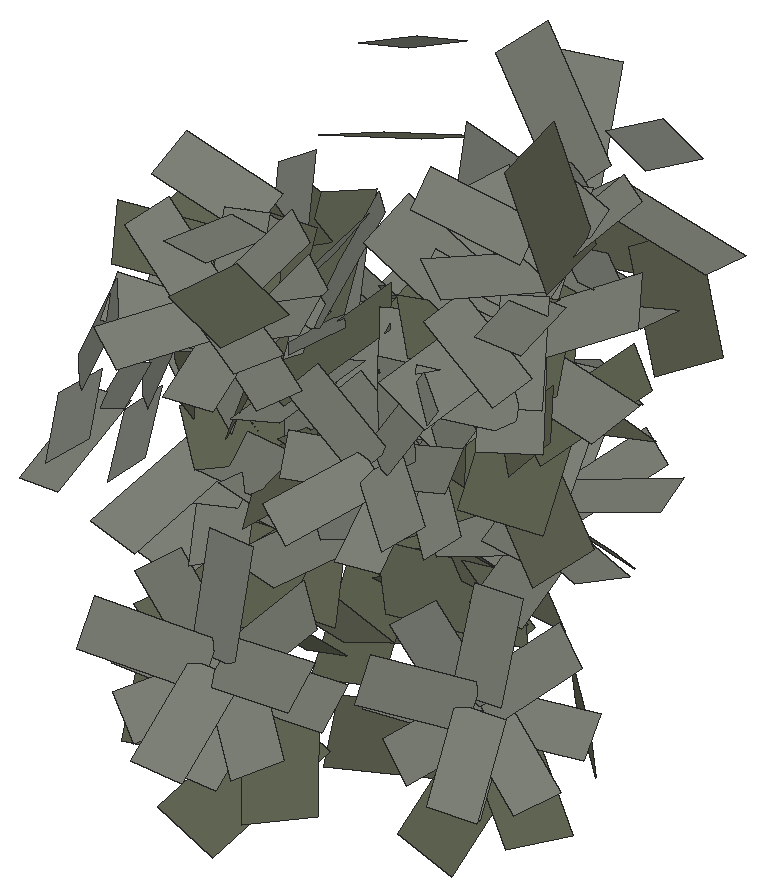
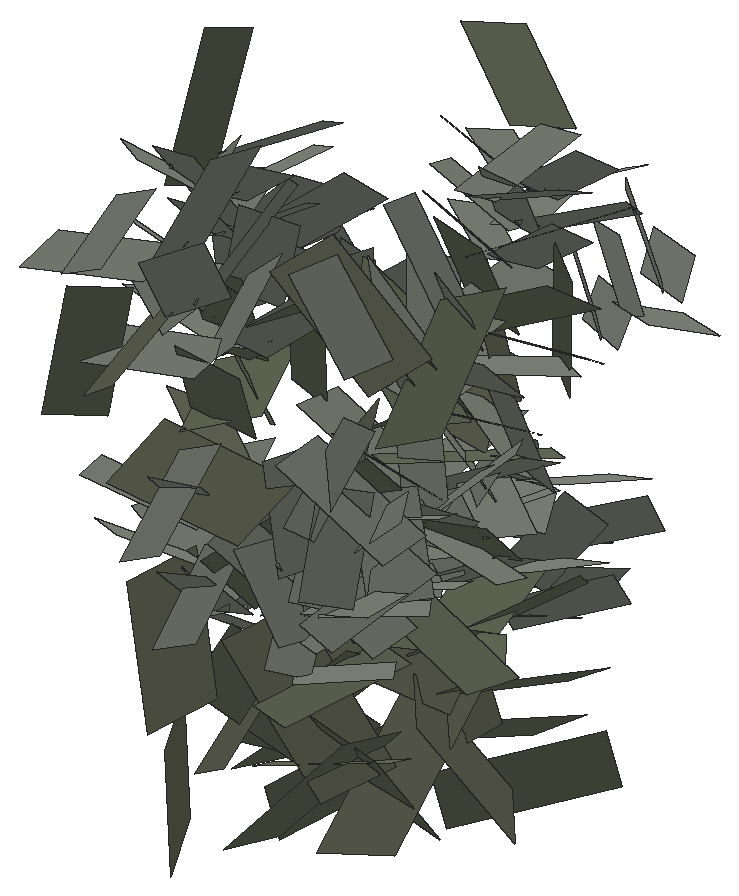
# SketchUp Ruby script. Lengths in inches.
U = 1.inch
M = Sketchup.active_model
def pt(a) = Geom::Point3d.new(a.map { |v| v * U })
def face(e, loops, mat)
  f = e.add_face(loops[0].map { |a| pt(a) })
  loops[1..].each { |l| e.add_face(l.map { |a| pt(a) }).erase! }
  f.material = f.back_material = mat if mat
  f
end
# faces: each face lists its corners as indices into pts; further lists are holes
def faces(e, pts, list, mat = nil) = list.each { |f| face(e, (f[0].is_a?(Array) ? f : [f]).map { |l| l.map { |i| pts[i] } }, mat) }
# xy, xz, yz: faces in a plane at the given z, y or x. An outline is a flat list of corners, or four numbers for a rectangle; further outlines are holes
def ring(l) = l.size == 4 ? [[l[0], l[1]], [l[2], l[1]], [l[2], l[3]], [l[0], l[3]]] : l.each_slice(2).to_a
def flat(e, list, mat, &to3) = list.each { |f| face(e, (f[0].is_a?(Array) ? f : [f]).map { |l| ring(l).map { |u, v| to3.(u, v) } }, mat) }
def xy(e, z, list, mat = nil) = flat(e, list, mat) { |x, y| [x, y, z] }
def xz(e, y, list, mat = nil) = flat(e, list, mat) { |x, z| [x, y, z] }
def yz(e, x, list, mat = nil) = flat(e, list, mat) { |y, z| [x, y, z] }
def lines(e, pts, list) = list.each { |a, b| e.add_line(pt(pts[a]), pt(pts[b])) }
# prism: a flat outline (further loops are holes) pulled along v
def prism(e, loops, v, mat = nil)
  f = face(e, loops, mat); d = Geom::Vector3d.new(v.map { |x| x * U })
  f.pushpull(f.normal.samedirection?(d) ? d.length : -d.length)
end
def box(e, o, s, mat = nil) = prism(e, [[o, [o[0] + s[0], o[1], o[2]], [o[0] + s[0], o[1] + s[1], o[2]], [o[0], o[1] + s[1], o[2]]]], [0, 0, s[2]], mat)
def at(x, y, z, deg = 0) = Geom::Transformation.translation(pt([x, y, z])) * Geom::Transformation.rotation(ORIGIN, Z_AXIS, deg.degrees)
def axes(o, x, y, z) = Geom::Transformation.new([*x, 0, *y, 0, *z, 0, *pt(o).to_a, 1])
def part(name) = M.definitions.add(name)
# library, detail: a bought-in or finely detailed component or shape, given as its bounding box
def library(name, o, s) = part(name).tap { |d| box(d.entities, o, s) }
def detail(e, o, s) = box(e.add_group.entities, o, s)
def put(e, d, t, mat = nil) = e.add_instance(d, t).tap { |i| i.material = mat if mat }
def group(e, t, mat = nil) = e.add_group.tap { |g| g.transformation = t; g.material = mat if mat }.entities
root = M.entities
M.materials.add("viburnumblaasdfas0df1w06d").color = [98, 102, 84]
M.materials.add("viburnumbladsadfasdfad0w122").color = [125, 129, 119]
c1 = part("Component\#315")
p = [[0.25,0,0],[2.05,0.01,0.35],[1.81,4.2,1.66],[0,4.19,1.3125]]
faces(c1.entities,p,[[0,1,2,3]],"viburnumbladsadfasdfad0w122")
c2 = part("viburnumblad2")
put(c2.entities,c1,axes([-19.23,-4.49,-32.18],[83.35428,0,0],[0,79.38502,0],[0,0,83.35428]))
c3 = part("Component\#314")
p = [[0.14,0,0],[2.58,0.05,0.25],[2.44,5.11,2.64],[0,5.05,2.39]]
faces(c3.entities,p,[[0,1,2,3]],"viburnumblaasdfas0df1w06d")
c4 = part("viburnumblad1\#2")
put(c4.entities,c3,axes([-37.25,6.23,19.31],[75.98784,0,0],[0,65.50676,0],[0,0,75.98784]))
put(root,c2,axes([1229.08,191.18,23.91],[-0.00766,-0.00322,-0.00823],[0.00764,-0.00813,-0.00386],[-0.0046,-0.00755,0.00633]))
put(root,c2,axes([1229.875,191.74,22.7],[-0.01118,0.00278,-0.00257],[-0.00011,-0.00839,-0.00838],[-0.00365,-0.00753,0.00688]))
put(root,c4,axes([1233.54,192.86,28.38],[-0.00662,-0.01127,-0.00498],[0.01432,-0.00702,-0.0031],[-0.00011,-0.00548,0.01154]))
put(root,c2,axes([1233.59,192.42,26.27],[-0.00995,0.00489,0.00397],[-0.00607,-0.00954,-0.00338],[0.0019,-0.00477,0.00949]))
put(root,c2,axes([1233.79,193.03,12.62],[-0.01241,-0.00141,0.00136],[-0.00002,-0.00862,-0.00914],[0.00196,-0.00903,0.00851]))
put(root,c2,axes([1227.68,191.68,23.79],[0.00814,-0.00715,-0.0046],[0.00716,0.00216,0.00888],[-0.00455,-0.00881,0.00477]))
put(root,c2,axes([1228.74,192.77,23.34],[0.00034,-0.00733,-0.00907],[0.00978,-0.00348,0.00299],[-0.00497,-0.00808,0.00546]))
put(root,c2,axes([1229.97,193.27,22.62],[-0.00655,-0.0022,-0.00816],[0.00764,-0.00813,-0.00386],[-0.0054,-0.00785,0.00541]))
put(root,c2,axes([1233.84,193.93,25.53],[-0.01146,-0.00283,-0.00038],[0.00275,-0.01049,-0.00491],[0.00082,-0.00467,0.00968]))
put(root,c2,axes([1233.51,193.6875,27.03],[-0.00626,-0.00889,-0.00451],[0.01001,-0.00557,-0.00285],[-0.00007,-0.00526,0.00943]))
put(root,c2,axes([1232.49,192.34,12.02],[0.00026,0.00745,0.01011],[-0.01208,-0.00262,0.00224],[0.00344,-0.00977,0.00711]))
put(root,c2,axes([1233.23,193.92,11.1875],[-0.00859,0.00427,0.00811],[-0.00794,-0.00683,-0.00482],[0.00302,-0.00917,0.00803]))
put(root,c2,axes([1232.85,192.9,25.04],[-0.00261,0.00974,0.006],[-0.01123,-0.00353,0.00072],[0.00254,-0.00551,0.00899]))
put(root,c2,axes([1232.92,193.69,13.76],[-0.00026,-0.00745,-0.01011],[0.01255,0.00018,-0.00046],[0.00042,-0.01011,0.00745]))
put(root,c2,axes([1233.14,194.77,12.4],[-0.00896,-0.00627,-0.00619],[0.0092,-0.00573,-0.00751],[0.00088,-0.00942,0.00827]))
put(root,c2,axes([1228.8,193.73,22.42],[0.0085,-0.00746,-0.0048],[0.00645,0.00195,0.00799],[-0.00455,-0.00881,0.00477]))
put(root,c2,axes([1232.1,192.27,26.35],[0.00626,0.00889,0.00451],[-0.00973,0.00413,0.00504],[0.00235,-0.00645,0.00846]))
put(root,c2,axes([1233.23,195.2,24.93],[-0.00572,-0.00761,-0.00506],[0.01001,-0.00557,-0.00285],[-0.00075,-0.00619,0.00889]))
put(root,c2,axes([1233.15,195.37,10.67],[-0.01296,-0.00148,0.00142],[-0.00002,-0.00776,-0.00823],[0.00196,-0.00903,0.00851]))
put(root,c2,axes([1231.62,193,13.17],[0.01241,0.00141,-0.00136],[0.00049,0.00618,0.01093],[0.0019,-0.01085,0.00605]))
put(root,c2,axes([1238.62,194.75,20.89],[-0.00871,0.00384,0.00541],[-0.00663,-0.00614,-0.00616],[0.00084,-0.00787,0.00624]))
put(root,c2,axes([1232.43,194.64,26.07],[0.00261,-0.00974,-0.006],[0.01057,0.00192,0.00135],[-0.00026,-0.0062,0.0089]))
put(root,c2,axes([1238.67,195.56,22],[-0.00668,-0.00514,-0.00687],[0.00865,-0.00485,-0.0047],[-0.00103,-0.00803,0.00606]))
put(root,c2,axes([1231.48,193.69,11.4],[0.00896,0.00627,0.00619],[-0.00837,0.00305,0.00903],[0.00298,-0.01046,0.00629]))
put(root,c2,axes([1232.03,193.55,27.11],[0.00995,-0.00489,-0.00397],[0.00635,0.0081,0.00558],[0.00038,-0.00694,0.0084]))
put(root,c2,axes([1232.09,194.68,10.17],[-0.00011,0.00779,0.00854],[-0.01208,-0.00262,0.00224],[0.00345,-0.0089,0.00816]))
put(root,c2,axes([1233.05,196.87,28.49],[-0.01199,0.00073,-0.00108],[-0.00063,-0.01339,-0.00213],[-0.00123,-0.0019,0.01236]))
put(root,c2,axes([1239.06,196.29,20.8125],[-0.01089,-0.00092,-0.00104],[0.00144,-0.00742,-0.00803],[-0.00015,-0.00772,0.00646]))
put(root,c2,axes([1231.75,194.66,12.66],[0.00859,-0.00427,-0.00811],[0.00913,0.005,0.00703],[0.00084,-0.0107,0.00653]))
put(root,c2,axes([1232.17,193.83,24.1],[0.00601,0.00853,0.00433],[-0.01051,0.00446,0.00545],[0.00235,-0.00645,0.00846]))
put(root,c2,axes([1231.79,193.55,25.51],[0.01146,0.00283,0.00038],[-0.00257,0.0094,0.00741],[0.00146,-0.00704,0.00821]))
put(root,c2,axes([1230.12,196.91,17.89],[-0.01312,0.00207,0.00149],[-0.00255,-0.01047,-0.0079],[-0.00005,-0.00804,0.01068]))
put(root,c2,axes([1232.14,196.01,11.74],[-0.00025,-0.00716,-0.0097],[0.01356,0.0002,-0.00049],[0.00042,-0.01011,0.00745]))
put(root,c2,axes([1237.23,194.77,20.95],[0.00668,0.00514,0.00687],[-0.00864,0.00277,0.00603],[0.00109,-0.00897,0.00475]))
put(root,c4,axes([1232.7,198.28,9.32],[-0.01126,-0.00753,-0.00255],[0.00827,-0.00884,-0.01044],[0.00351,-0.00867,0.01012]))
put(root,c4,axes([1229.32,195.73,20.55],[0.01089,-0.00679,0.00142],[0.00218,0.00667,0.0129],[-0.00665,-0.00902,0.00468]))
put(root,c4,axes([1232.75,196.73,25.15],[-0.0066,0.01089,0.00527],[-0.0139,-0.00777,-0.00135],[0.00164,-0.00514,0.01268]))
put(root,c2,axes([1238.04,195.71,20.04],[-0.00143,0.00635,0.00868],[-0.0108,-0.00196,-0.00037],[0.00136,-0.00839,0.00553]))
put(root,c2,axes([1237.29,195.58,22.05],[0.00871,-0.00384,-0.00541],[0.00664,0.00406,0.00749],[-0.00079,-0.00912,0.00457]))
put(root,c2,axes([1231.97,195.07,24.9],[0.01038,-0.0051,-0.00415],[0.00572,0.00729,0.00502],[0.00038,-0.00694,0.0084]))
put(root,c4,axes([1232.74,198.97,19.44],[-0.00918,-0.00626,-0.00848],[0.01129,-0.01094,-0.00412],[-0.00395,-0.00772,0.00939]))
put(root,c4,axes([1230.57,197.7,20.49],[0.00428,-0.01029,-0.00658],[0.01194,-0.00078,0.00879],[-0.00649,-0.00737,0.00685]))
put(root,c2,axes([1237.83,196.86,21.56],[0.00143,-0.00635,-0.00868],[0.00992,-0.00012,0.00155],[-0.0013,-0.00861,0.00528]))
put(root,c4,axes([1232.6,199.28,6.97],[-0.01186,-0.00066,0.00699],[-0.00532,-0.01121,-0.01007],[0.00532,-0.0098,0.0081]))
put(root,c2,axes([1232.3,198.48,24.74],[-0.01244,-0.00019,-0.00567],[0.00199,-0.01294,-0.00394],[-0.00531,-0.00441,0.0118]))
put(root,c2,axes([1238.68,197.67,20.78],[-0.00601,-0.0039,-0.00689],[0.00865,-0.00485,-0.0047],[-0.00175,-0.00854,0.00529]))
put(root,c2,axes([1229.42,198.03,18.94],[-0.00252,-0.00942,-0.00914],[0.01298,-0.00318,-0.00031],[-0.00196,-0.00893,0.00974]))
put(root,c2,axes([1229.9,198.8,17.3125],[-0.01106,-0.0052,-0.00541],[0.00776,-0.00965,-0.0066],[-0.00127,-0.0082,0.01048]))
put(root,c2,axes([1231.8,195.9375,28.14],[0.00044,0.0126,0.00361],[-0.0113,0.00031,0.00032],[0.00024,-0.00347,0.01207]))
put(root,c2,axes([1240.93,198.61,11.125],[-0.01026,-0.00498,0.00256],[0.0015,-0.00759,-0.00876],[0.0054,-0.00736,0.0073]))
put(root,c2,axes([1239.93,197.61,10.69],[-0.00083,0.00664,0.00958],[-0.0095,-0.00594,0.0033],[0.00675,-0.00756,0.00582]))
put(root,c2,axes([1237.125,196.21,20.71],[0.01089,0.00092,0.00104],[-0.00149,0.00552,0.00975],[0.0002,-0.00927,0.00435]))
put(root,c4,axes([1231.34,196.125,22.41],[0.01287,-0.00107,0.00071],[0.00034,0.01171,0.00907],[-0.00141,-0.0079,0.00892]))
put(root,c4,axes([1232.83,199.58,19.46],[-0.00628,-0.01206,-0.00336],[0.01448,-0.00668,-0.00311],[0.00091,-0.00388,0.01211]))
put(root,c2,axes([1233.52,199.6,17.84],[-0.01428,0.00021,0.00102],[-0.00037,-0.01414,-0.00224],[0.00098,-0.00226,0.01411]))
put(root,c2,axes([1230,199.08,15.39],[-0.0137,0.00216,0.00156],[-0.00229,-0.00943,-0.00711],[-0.00005,-0.00804,0.01068]))
put(root,c2,axes([1237.56,196.9375,19.61],[0.00642,0.00493,0.0066],[-0.00933,0.00299,0.00651],[0.00109,-0.00897,0.00475]))
put(root,c2,axes([1241.58,198.21,22.68],[-0.00449,0.00779,0.00619],[-0.00867,-0.00648,0.00177],[0.0049,-0.00408,0.00781]))
put(root,c2,axes([1232.61,198.76,22.875],[-0.01065,0.00857,-0.00023],[-0.00787,-0.00997,-0.00669],[-0.00415,-0.00484,0.01209]))
put(root,c2,axes([1240,199.22,9.9],[-0.00784,0.00117,0.00859],[-0.00546,-0.0084,-0.00383],[0.00631,-0.00716,0.00674]))
put(root,c2,axes([1237.49,197.72,20.74],[0.00909,-0.00401,-0.00564],[0.00597,0.00365,0.00674],[-0.00079,-0.00912,0.00457]))
put(root,c2,axes([1240.67,200,24.8],[-0.01366,0.00095,0.00535],[-0.00336,-0.01286,-0.00628],[0.00428,-0.00706,0.01216]))
put(root,c2,axes([1233.24,200.25,21.93],[-0.01194,-0.00018,-0.00545],[0.00215,-0.01397,-0.00426],[-0.00531,-0.00441,0.0118]))
put(root,c2,axes([1232.42,200.14,23.55],[-0.00694,-0.00883,-0.00779],[0.00996,-0.00923,0.0016],[-0.00629,-0.00487,0.01112]))
put(root,c4,axes([1231.67,197.14,22.86],[0.0051,0.011,0.00655],[-0.01483,0.00551,0.0023],[-0.00067,-0.00681,0.01196]))
put(root,c2,axes([1241.27,197.43,23.96],[0.00334,0.0097,0.00381],[-0.00915,0.00071,0.00588],[0.00496,-0.00497,0.00731]))
put(root,c2,axes([1231.21,197.57,23.76],[-0.00263,0.0123,0.00535],[-0.01296,-0.00091,-0.00426],[-0.00348,-0.00589,0.01184]))
put(root,c4,axes([1231.57,198.18,21.39],[0.0077,-0.00971,-0.00377],[0.01191,0.00736,0.00523],[-0.00177,-0.00557,0.01033]))
put(root,c2,axes([1233,200.9,14.51],[-0.01371,0.0002,0.00098],[-0.0004,-0.01527,-0.00242],[0.00098,-0.00226,0.01411]))
put(root,c4,axes([1230.25,201.88,13.42],[-0.01365,-0.00518,-0.0014],[0.0059,-0.01311,-0.00908],[0.00168,-0.00777,0.01232]))
put(root,c2,axes([1227.89,197.56,18.43],[0.01312,-0.00207,-0.00149],[0.00246,0.00822,0.01025],[-0.00067,-0.01033,0.00845]))
put(root,c2,axes([1232.86,199.58,15.95],[-0.00976,0.00988,0.00351],[-0.01076,-0.01049,-0.00039],[0.00219,-0.00277,0.01388]))
put(root,c2,axes([1231.125,199.74,24.875],[0.00263,-0.0123,-0.00535],[0.01173,-0.00054,0.007],[-0.00651,-0.00594,0.01045]))
put(root,c4,axes([1230.91,200.64,4.82],[-0.00011,0.00616,0.01357],[-0.0165,-0.00475,0.00202],[0.00445,-0.01294,0.00591]))
put(root,c2,axes([1229.17,200.2,16.37],[-0.00242,-0.00904,-0.00878],[0.01402,-0.00344,-0.00033],[-0.00196,-0.00893,0.00974]))
put(root,c2,axes([1233.06,201.11,16.41],[-0.01044,-0.00958,-0.00206],[0.0098,-0.01029,-0.00181],[-0.00027,-0.00273,0.01406]))
put(root,c2,axes([1239.8125,199.95,11.06],[-0.00667,-0.00821,-0.00496],[0.00888,-0.00228,-0.00816],[0.00454,-0.00802,0.00718]))
put(root,c4,axes([1234.13,200.6875,18.41],[-0.01024,0.01003,0.00441],[-0.01249,-0.0094,-0.00763],[-0.00202,-0.00765,0.01274]))
put(root,c2,axes([1239.44,200.47,9.49],[-0.01071,-0.0052,0.00268],[0.00135,-0.00683,-0.00788],[0.0054,-0.00736,0.0073]))
put(root,c2,axes([1238.57,198.5,10.28],[0.00667,0.00821,0.00496],[-0.00717,0.00016,0.00937],[0.00645,-0.00831,0.00509]))
put(root,c2,axes([1238.66,199.55,9.12],[-0.00143,0.00682,0.00818],[-0.0095,-0.00594,0.0033],[0.00662,-0.0068,0.00682]))
put(root,c2,axes([1239.1,197.93,11.87],[0.01026,0.00498,-0.00256],[-0.00015,0.00559,0.01026],[0.0056,-0.00897,0.00496]))
put(root,c2,axes([1228.44,199.11,17.59],[0.00749,-0.00812,-0.00752],[0.01093,0.00403,0.00654],[-0.00171,-0.00982,0.0089]))
put(root,c4,axes([1232.05,200.74,10.8],[-0.00702,0.01204,0.00725],[-0.01547,-0.00958,0.00093],[0.00442,-0.0058,0.01392]))
put(root,c2,axes([1241.13,200.64,27.13],[-0.00997,0.00542,0.0028],[-0.00605,-0.01063,-0.00096],[0.002,-0.00216,0.01131]))
put(root,c2,axes([1232.01,198.62,17.65],[0.00048,0.01376,0.00394],[-0.01406,-0.00028,0.00269],[0.00266,-0.00396,0.0135]))
put(root,c2,axes([1240.6,198.82,21.93],[0.0032,0.00932,0.00366],[-0.00988,0.00076,0.00635],[0.00496,-0.00497,0.00731]))
put(root,c4,axes([1237.13,199.64,19.03],[0.0117,-0.0027,-0.00014],[0.00141,0.00653,0.01192],[-0.00257,-0.00994,0.00471]))
put(root,c2,axes([1239.97,201.94,24.04],[-0.01238,-0.00774,-0.00167],[0.00772,-0.01057,-0.00819],[0.00296,-0.0074,0.01235]))
put(root,c4,axes([1230.33,202.48,10.75],[-0.01218,0.00376,0.00725],[-0.00872,-0.0119,-0.00846],[0.0032,-0.00977,0.01045]))
put(root,c2,axes([1240.97,201.76,26],[-0.01081,-0.00296,0.00035],[0.0032,-0.01197,-0.0024],[0.00093,-0.00205,0.01147]))
put(root,c2,axes([1239.64,200.55,23.07],[-0.00693,0.00909,0.00924],[-0.01085,-0.00802,-0.00026],[0.00532,-0.00757,0.01142]))
put(root,c4,axes([1240.36,201.55,22.94],[-0.0084,0.0076,0.00599],[-0.00998,-0.01102,-0.00002],[0.00443,-0.00403,0.01133]))
put(root,c4,axes([1229.4375,201.54,8.47],[-0.00936,-0.00715,0.0061],[0.00985,-0.01174,0.00135],[0.00403,0.00472,0.01172]))
put(root,c2,axes([1240.64,199.63,28.47],[-0.00283,0.01075,0.0036],[-0.01102,-0.00348,0.00171],[0.00265,-0.00298,0.01098]))
put(root,c2,axes([1238.98,199.24,24.79],[0.00385,0.0119,0.00772],[-0.01309,-0.0001,0.00669],[0.00547,-0.00863,0.01057]))
put(root,c2,axes([1232.23,199.2,20.97],[-0.00274,0.01284,0.00559],[-0.01166,-0.00082,-0.00384],[-0.00348,-0.00589,0.01184]))
put(root,c2,axes([1240.52,198.46,23.26],[0.0092,0.00594,-0.0008],[-0.00419,0.00749,0.00747],[0.00433,-0.00576,0.00715]))
put(root,c2,axes([1232.53,201.03,18.32],[-0.00048,-0.01376,-0.00394],[0.01429,-0.00069,0.00066],[-0.00082,-0.00391,0.01375]))
put(root,c2,axes([1239.48,201.96,21.96],[-0.01426,0.00099,0.00559],[-0.00302,-0.01157,-0.00566],[0.00428,-0.00706,0.01216]))
put(root,c2,axes([1231.07,201.39,16.84],[-0.01065,0.00247,0.00234],[-0.00174,-0.01065,0.00331],[0.00294,0.00276,0.01043]))
put(root,c2,axes([1227.85,201.9,18.53],[-0.00829,-0.0091,-0.00248],[0.00914,-0.00728,-0.00415],[0.002,-0.00468,0.01099]))
put(root,c2,axes([1231.18,198.63,22.14],[0.00694,0.00883,0.00779],[-0.01027,0.00714,0.00105],[-0.0037,-0.00696,0.01117]))
put(root,c2,axes([1238.66,199.43,11.45],[0.00784,-0.00117,-0.00859],[0.00729,0.00715,0.00568],[0.00468,-0.00917,0.00553]))
put(root,c2,axes([1230.64,202.04,15.56],[-0.00842,-0.00565,0.00174],[0.00635,-0.00914,0.00106],[0.00096,0.00194,0.01097]))
put(root,c2,axes([1230.03,198.83,23.9],[0.01244,0.00019,0.00567],[-0.00322,0.01148,0.00668],[-0.00467,-0.00741,0.01049]))
put(root,c2,axes([1231.24,202.29,18.16],[-0.009,-0.00589,0.00306],[0.00635,-0.00914,0.00106],[0.00195,0.00259,0.0107]))
put(root,c2,axes([1231.57,199.78,14.33],[0.00051,0.01437,0.00412],[-0.01266,-0.00025,0.00242],[0.00266,-0.00396,0.0135]))
put(root,c4,axes([1241.1,200.79,26.83],[0.00008,0.01316,0.00435],[-0.00745,-0.00443,0.01354],[0.01228,-0.00208,0.00607]))
put(root,c4,axes([1238.02,202.9,8.4],[-0.00788,-0.01001,-0.0014],[0.00865,-0.00529,-0.01087],[0.00682,-0.00657,0.00863]))
put(root,c4,axes([1237.36,203.75,6.27],[-0.00935,-0.00415,0.00773],[-0.00246,-0.01147,-0.00913],[0.00851,-0.00702,0.00652]))
put(root,c2,axes([1238.49,200.74,10.61],[0.00079,-0.00637,-0.0092],[0.01172,0.00425,-0.00193],[0.00425,-0.00877,0.00644]))
put(root,c2,axes([1240.11,200.57,25.77],[-0.00295,0.01122,0.00376],[-0.00992,-0.00313,0.00154],[0.00265,-0.00298,0.01098]))
put(root,c4,axes([1237.63,201.75,18.92],[0.00605,-0.00776,-0.00693],[0.01168,0.0029,0.00677],[-0.00267,-0.00844,0.00676]))
put(root,c2,axes([1230.76,201,18.45],[-0.00607,0.00939,0.00026],[-0.0086,-0.00567,0.00435],[0.00378,0.00216,0.0103]))
put(root,c2,axes([1230.79,200.35,22.93],[0.01065,-0.00857,0.00023],[0.00633,0.00812,0.0092],[-0.00584,-0.00699,0.01019]))
put(root,c4,axes([1238.74,204.72,19.48],[-0.01393,-0.0074,0.00333],[0.00558,-0.01491,-0.00981],[0.00654,-0.00631,0.01332]))
put(root,c4,axes([1239.02,203.52,17.76],[-0.00713,-0.00827,-0.00706],[0.01264,-0.00623,-0.00545],[-0.00006,-0.00799,0.0088]))
put(root,c4,axes([1231.02,199.13,20.64],[0.01421,-0.00084,0.00442],[-0.0012,0.01582,0.00687],[-0.00438,-0.00595,0.01294]))
put(root,c2,axes([1231.18,199.48,16.01],[0.01044,0.00958,0.00206],[-0.00879,0.00856,0.00474],[0.00211,-0.00514,0.0132]))
put(root,c2,axes([1239.83,200.18,27.125],[0.00596,0.00978,0.00229],[-0.00894,0.00456,0.00379],[0.00249,-0.00402,0.01069]))
put(root,c4,axes([1237.97,204.96,16.59],[-0.01126,0.00378,0.01091],[-0.00977,-0.0152,-0.00482],[0.00789,-0.0086,0.01113]))
put(root,c4,axes([1239.03,201.58,20.96],[0.00193,0.01121,0.0059],[-0.01433,0.00039,0.00396],[0.00283,-0.0062,0.01085]))
put(root,c4,axes([1233.78,201.4375,15.75],[0.00121,0.01104,0.01007],[-0.01675,0.00403,-0.00241],[-0.00386,-0.00953,0.01091]))
put(root,c2,axes([1238.1,201.18,21.99],[0.00298,0.01174,0.00601],[-0.01309,-0.0001,0.00669],[0.00586,-0.00729,0.01134]))
put(root,c4,axes([1238.99,200.6,20.54],[0.01164,0.00293,-0.00079],[-0.00215,0.01041,0.00877],[0.00216,-0.00738,0.00809]))
put(root,c2,axes([1230.21,202.71,16.85],[-0.00207,-0.01081,0.00198],[0.01001,-0.00209,-0.00093],[0.00139,0.00174,0.01096]))
put(root,c2,axes([1238.72,203.22,23.11],[-0.0037,-0.01142,-0.00741],[0.01514,-0.00214,-0.00425],[0.00214,-0.0084,0.01187]))
put(root,c2,axes([1231.15,200.1875,21.14],[0.01184,0.00091,0.00415],[-0.00322,0.01148,0.00668],[-0.0033,-0.00735,0.01104]))
put(root,c2,axes([1238.38,200.53,25.98],[0.01366,-0.00095,-0.00535],[0.00429,0.01077,0.00904],[0.00334,-0.00996,0.01028]))
put(root,c2,axes([1239.33,204.3,16.22],[-0.01242,-0.00411,0.00252],[0.00364,-0.01255,-0.00256],[0.00316,-0.0017,0.01283]))
put(root,c2,axes([1231.02,200.05,18.14],[0.01428,-0.00021,-0.00102],[0.00059,0.01317,0.00559],[0.00086,-0.00561,0.01315]))
put(root,c4,axes([1235.23,204.4375,4.53],[-0.00036,0.00539,0.01277],[-0.01275,-0.00915,0.0035],[0.00843,-0.01005,0.00448]))
put(root,c2,axes([1226.58,202.75,17.48],[0.00038,-0.01114,-0.00561],[0.01301,0.00109,-0.00087],[0.0016,-0.0057,0.01058]))
put(root,c2,axes([1231.25,201.41,16.61],[0.00976,-0.00988,-0.00351],[0.01058,0.00912,0.00376],[-0.00035,-0.00511,0.01338]))
put(root,c4,axes([1227.07,201.29,5.83],[0.01021,-0.01095,0.0021],[0.01009,0.01114,0.00903],[-0.00698,-0.00405,0.01279]))
put(root,c2,axes([1237.73,200.66,23.86],[0.01238,0.00774,0.00167],[-0.00648,0.00805,0.01066],[0.00465,-0.00962,0.01009]))
put(root,c2,axes([1238.48,202.14,24.74],[0.00693,-0.00909,-0.00924],[0.01276,0.00664,0.00304],[0.0023,-0.00946,0.01102]))
put(root,c2,axes([1238.54,204.09,14.55],[-0.01106,0.00576,0.00468],[-0.00631,-0.01247,0.00042],[0.00435,-0.00178,0.01246]))
put(root,c4,axes([1228.69,202.36,10.95],[0.00308,-0.0114,0.00333],[0.01375,0.00318,-0.00182],[0.00071,0.00361,0.0117]))
put(root,c4,axes([1229.13,205.8,22.59],[-0.01489,-0.00148,0.00524],[0.00198,-0.01828,0.00047],[0.00517,0.00094,0.01496]))
put(root,c4,axes([1236.89,204.87,9.93],[-0.00888,0.00849,0.00791],[-0.01054,-0.01309,0.0022],[0.00721,-0.00377,0.01214]))
put(root,c2,axes([1239.44,201.6875,27.66],[0.00997,-0.00542,-0.0028],[0.00614,0.00939,0.00366],[0.00055,-0.00455,0.01075]))
put(root,c2,axes([1229.51,202.43,15.7],[0.00633,-0.0098,-0.00027],[0.00833,0.00542,-0.00155],[0.00159,0.00072,0.01104]))
put(root,c2,axes([1238.1,205.3,13.25],[-0.01192,-0.00395,0.00242],[0.00393,-0.01356,-0.00276],[0.00316,-0.0017,0.01283]))
put(root,c2,axes([1230.67,200.93,14.84],[0.01298,0.00037,-0.00224],[0.00059,0.01317,0.00559],[0.0024,-0.0056,0.01296]))
put(root,c2,axes([1239.14,201.25,26.1875],[0.01014,0.00329,-0.00138],[-0.00265,0.01026,0.00493],[0.00283,-0.00431,0.01049]))
put(root,c2,axes([1238.28,202.99,16.18],[-0.00323,0.01225,0.0041],[-0.01189,-0.00447,0.00401],[0.00507,-0.00269,0.01202]))
put(root,c4,axes([1232.12,206.56,15.36],[-0.01205,-0.00086,0.01408],[0.00278,-0.02131,0.00108],[0.0139,0.00242,0.01204]))
put(root,c2,axes([1229.125,201.09,15.94],[0.00864,0.00566,-0.00294],[-0.00615,0.01026,0.00169],[0.00342,0.0003,0.01064]))
put(root,c4,axes([1238.46,202.48,19.66],[0.00918,-0.00623,-0.00469],[0.00881,0.01006,0.00379],[0.00131,-0.00544,0.00952]))
put(root,c2,axes([1229.96,202.83,18.4],[0.00607,-0.00939,-0.00026],[0.00926,0.00603,-0.00173],[0.00159,0.00072,0.01104]))
put(root,c4,axes([1225.9,204.79,13.5],[-0.00229,-0.01326,-0.00295],[0.0155,-0.0021,-0.00237],[0.00206,-0.00324,0.01267]))
put(root,c2,axes([1229.48,201.54,18.7],[0.009,0.00589,-0.00306],[-0.00569,0.0095,0.00156],[0.00342,0.0003,0.01064]))
put(root,c2,axes([1229.21,201.93,17.22],[0.01065,-0.00247,-0.00234],[0.00251,0.01145,-0.00069],[0.00243,0.00013,0.01091]))
put(root,c2,axes([1238.31,205.5,15.01],[-0.0065,-0.01157,-0.00112],[0.01142,-0.00611,-0.00313],[0.00221,-0.00249,0.0129]))
put(root,c2,axes([1239.68,206.1,26.92],[-0.01234,0.00028,0.00961],[0.00075,-0.01555,0.00142],[0.00958,0.00158,0.01226]))
put(root,c2,axes([1237.49,206.26,23.89],[-0.01223,0.0001,0.00757],[0.00075,-0.01555,0.00142],[0.00819,0.0016,0.01322]))
put(root,c4,axes([1230.46,207.41,6.45],[-0.01776,-0.00139,0.00308],[0.00179,-0.02087,0.00087],[0.003,0.001,0.0178]))
put(root,c4,axes([1228.36,201.79,13.14],[0.01107,-0.00525,0.00049],[0.00612,0.01279,-0.0012],[0,0.00115,0.01221]))
put(root,c2,axes([1237.17,203.88,13.2],[-0.00337,0.01279,0.00428],[-0.0107,-0.00403,0.00361],[0.00507,-0.00269,0.01202]))
put(root,c2,axes([1238.16,205.18,25.57],[-0.00842,0.01125,0.00685],[-0.00786,-0.01092,0.00827],[0.01063,0.001,0.01143]))
put(root,c4,axes([1235.05,204.74,7.9375],[0.0025,0.01316,0.00583],[-0.01545,-0.00015,0.00696],[0.00546,-0.00635,0.01198]))
put(root,c4,axes([1235.48,205.92,14.21],[0.00442,0.01183,0.01203],[-0.01827,-0.00182,0.0085],[0.00605,-0.01272,0.01028]))
put(root,c2,axes([1237.11,203.5,14.79],[0.0065,0.01157,0.00112],[-0.00968,0.00489,0.00566],[0.0049,-0.00389,0.01176]))
put(root,c2,axes([1238.09,205.27,16.82],[0.00323,-0.01225,-0.0041],[0.01276,0.00369,-0.00099],[0.00204,-0.00369,0.01263]))
put(root,c4,axes([1237.62,203.15,19.06],[0.01317,0.00353,0.00249],[-0.00497,0.01356,0.00706],[-0.00054,-0.00655,0.0122]))
put(root,c2,axes([1228.73,207.28,17.9],[-0.01077,-0.01069,-0.00135],[0.00977,-0.00996,0.00094],[-0.00168,-0.00022,0.01514]))
put(root,c2,axes([1238.19,207.39,25.54],[-0.00902,-0.01086,0.00673],[0.00875,-0.01029,-0.00487],[0.0085,0.00104,0.01308]))
put(root,c4,axes([1228.52,206.87,25.59],[-0.00484,-0.01365,0.00231],[0.016,-0.00575,-0.00049],[0.00117,0.00203,0.01447]))
put(root,c4,axes([1233.6,203.91,13.54],[0.01304,-0.00033,0.00964],[-0.00605,0.01553,0.00873],[-0.00811,-0.00915,0.01066]))
put(root,c4,axes([1229.17,203.4,6.07],[0.01682,-0.00022,0.00237],[-0.00091,0.01794,0.00812],[-0.00224,-0.00704,0.0153]))
put(root,c4,axes([1230.84,205.83,8.77],[-0.00166,-0.01224,0.00834],[0.01717,-0.00122,0.00163],[-0.00056,0.00844,0.01227]))
put(root,c2,axes([1237.04,203.95,16.78],[0.01242,0.00411,-0.00252],[-0.00277,0.01177,0.00559],[0.00395,-0.00468,0.01183]))
put(root,c2,axes([1238.38,205,27.91],[0.00042,0.01563,0.00009],[-0.01107,0.00024,0.01104],[0.01103,-0.00036,0.01108]))
put(root,c4,axes([1235.39,208.38,8.43],[-0.01278,0.00636,0.00656],[-0.00548,-0.01653,0.00535],[0.00782,0.00178,0.01351]))
put(root,c2,axes([1227.92,207.45,19.89],[0,-0.01516,-0.00154],[0.01507,-0.00022,0.00221],[-0.00223,-0.00152,0.015]))
put(root,c4,axes([1233.21,208.11,18.66],[-0.00321,-0.01557,0.00645],[0.01613,-0.00714,-0.00921],[0.00952,0.00374,0.01377]))
put(root,c2,axes([1232.27,208.1,17.97],[-0.01038,-0.0062,0.0034],[0.00714,-0.00931,0.00482],[0.00014,0.00586,0.01111]))
put(root,c2,axes([1232.34,207.75,19.83],[-0.01229,0.00259,0.00001],[-0.00225,-0.0107,0.00618],[0.00128,0.00604,0.01094]))
put(root,c2,axes([1236.64,207.61,24.4375],[-0.00044,-0.01632,-0.00009],[0.01207,-0.00029,-0.00723],[0.00803,-0.00029,0.01342]))
put(root,c2,axes([1236.67,205.22,15.4],[0.01106,-0.00576,-0.00468],[0.00696,0.01121,0.00265],[0.00276,-0.0046,0.01219]))
put(root,c2,axes([1228.24,207.63,16.125],[0,-0.01583,-0.00161],[0.01357,-0.0002,0.00199],[-0.00223,-0.00152,0.015]))
put(root,c2,axes([1231.55,208.24,16.15],[-0.01032,0.0026,-0.00299],[-0.00231,-0.01123,-0.0018],[-0.0033,-0.001,0.0105]))
put(root,c2,axes([1231.17,208.5,17.62],[-0.00856,-0.00558,-0.00422],[0.00556,-0.00947,0.00126],[-0.00425,-0.00115,0.01014]))
put(root,c4,axes([1235.9,208.89,4.82],[-0.00616,-0.00011,0.01357],[0.00475,-0.0165,0.00202],[0.01294,0.00445,0.00591]))
put(root,c4,axes([1232.73,208.7,12.23],[-0.011,0.00511,-0.00003],[-0.00581,-0.01252,-0.00271],[-0.00101,-0.0021,0.0119]))
put(root,c2,axes([1238.83,207.74,27.63],[-0.00042,-0.01563,-0.00009],[0.01341,-0.00032,-0.00803],[0.00803,-0.00029,0.01342]))
put(root,c2,axes([1231.73,206.71,18.58],[-0.007,0.00987,-0.00339],[-0.01018,-0.00558,0.00479],[0.00226,0.00542,0.01111]))
put(root,c2,axes([1236.1,204.625,13.8125],[0.01096,0.00423,-0.00348],[-0.00277,0.01177,0.00559],[0.00527,-0.00421,0.01149]))
put(root,c4,axes([1229.22,208.65,9.72],[-0.00613,-0.01546,0.00166],[0.01796,-0.00686,0.00247],[-0.00138,0.00232,0.01649]))
put(root,c2,axes([1230.72,207.25,17.18],[-0.00604,0.00926,-0.00001],[-0.00892,-0.00582,-0.00295],[-0.00247,-0.0016,0.01066]))
put(root,c2,axes([1230.34,208.96,17.18],[-0.01091,0.00229,-0.00461],[-0.00339,-0.01305,0.00154],[-0.00434,0.00249,0.01152]))
put(root,c2,axes([1231.74,209.17,14.97],[-0.00821,-0.00536,-0.00406],[0.00601,-0.01023,0.00136],[-0.00425,-0.00115,0.01014]))
put(root,c2,axes([1231.41,208.1,16.52],[-0.00213,-0.01089,0.00325],[0.01232,-0.002,0.0014],[-0.00076,0.00372,0.01198]))
put(root,c4,axes([1239.4,209.65,22.86],[-0.011,0.0051,0.00655],[-0.00551,-0.01483,0.0023],[0.00681,-0.00067,0.01196]))
put(root,c4,axes([1235.8,210.03,10.8],[-0.01204,-0.00702,0.00725],[0.00958,-0.01547,0.00093],[0.0058,0.00442,0.01392]))
put(root,c4,axes([1240.8125,207.3,20.55],[0.00679,0.01089,0.00142],[-0.00667,0.00218,0.0129],[0.00902,-0.00665,0.00468]))
put(root,c2,axes([1231.39,207.86,14.59],[-0.0063,0.00967,-0.00001],[-0.00803,-0.00524,-0.00265],[-0.00247,-0.0016,0.01066]))
put(root,c2,axes([1236.76,209.55,14.33],[-0.01437,0.00051,0.00412],[0.00025,-0.01266,0.00242],[0.00396,0.00266,0.0135]))
put(root,c2,axes([1230.97,206.2,17.18],[0.00229,0.01091,-0.00461],[-0.01305,0.00339,0.00154],[0.00249,0.00434,0.01152]))
put(root,c2,axes([1229.83,209.72,18.58],[-0.00987,-0.007,-0.00339],[0.00558,-0.01018,0.00479],[-0.00542,0.00226,0.01111]))
put(root,c4,axes([1233.14,207.15,6.07],[0.00022,0.01682,0.00237],[-0.01794,-0.00091,0.00812],[0.00704,-0.00224,0.0153]))
put(root,c2,axes([1237.92,209.99,17.65],[-0.01376,0.00048,0.00394],[0.00028,-0.01406,0.00269],[0.00396,0.00266,0.0135]))
put(root,c4,axes([1232.59,208.32,10],[-0.00341,0.01096,0.00392],[-0.01337,-0.00302,-0.00319],[-0.00164,-0.0045,0.01114]))
put(root,c2,axes([1236.6,205.52,26.79],[0.00902,0.01086,-0.00673],[-0.00719,0.01113,0.00831],[0.01056,-0.0017,0.01141]))
put(root,c2,axes([1240.6,209.78,28.14],[-0.0126,0.00044,0.00361],[-0.00031,-0.0113,0.00032],[0.00347,0.00024,0.01207]))
put(root,c2,axes([1227.97,209.625,28.15],[-0.00597,-0.01037,0.00113],[0.01154,-0.00613,0.0032],[-0.00222,0.00293,0.01099]))
put(root,c2,axes([1230.95,209.33,16.21],[-0.00178,-0.0105,-0.00298],[0.00981,-0.00286,0.00422],[-0.00478,-0.00196,0.00978]))
